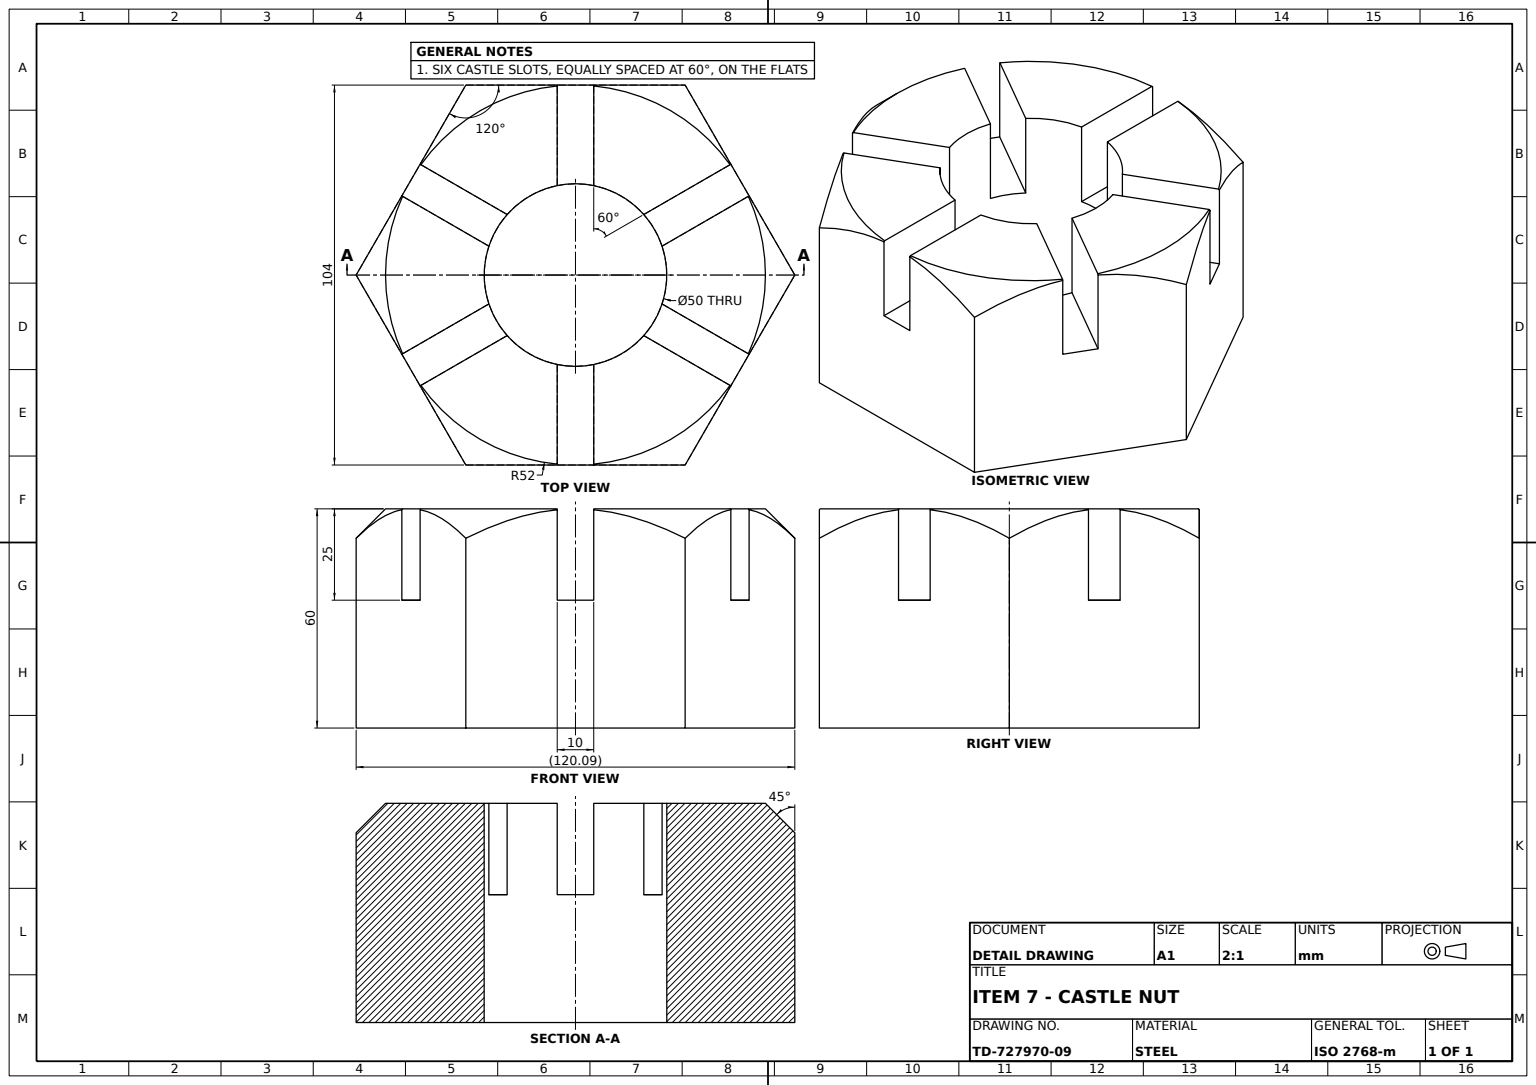
ISO-10303-21;
HEADER;
FILE_DESCRIPTION((''),'2;1');
FILE_NAME('','',(''),(''),'','','');
FILE_SCHEMA(('AUTOMOTIVE_DESIGN'));
ENDSEC;
DATA;
#1=APPLICATION_CONTEXT('');
#2=PRODUCT_CONTEXT('',#1,'mechanical');
#3=PRODUCT('','','',(#2));
#4=PRODUCT_DEFINITION_FORMATION('','',#3);
#5=PRODUCT_DEFINITION_CONTEXT('',#1,'design');
#6=PRODUCT_DEFINITION('','',#4,#5);
#7=PRODUCT_DEFINITION_SHAPE('','',#6);
#8=(LENGTH_UNIT()NAMED_UNIT(*)SI_UNIT(.MILLI.,.METRE.));
#9=(NAMED_UNIT(*)PLANE_ANGLE_UNIT()SI_UNIT($,.RADIAN.));
#10=(NAMED_UNIT(*)SI_UNIT($,.STERADIAN.)SOLID_ANGLE_UNIT());
#11=UNCERTAINTY_MEASURE_WITH_UNIT(LENGTH_MEASURE(1.E-05),#8,'distance_accuracy_value','');
#12=(GEOMETRIC_REPRESENTATION_CONTEXT(3)GLOBAL_UNCERTAINTY_ASSIGNED_CONTEXT((#11))GLOBAL_UNIT_ASSIGNED_CONTEXT((#8,#9,#10))REPRESENTATION_CONTEXT('',''));
#13=CARTESIAN_POINT('',(-23.713203,35.,-7.917322));
#14=VERTEX_POINT('',#13);
#15=CARTESIAN_POINT('',(-23.713203,60.,-7.917322));
#16=VERTEX_POINT('',#15);
#17=DIRECTION('',(0.,1.,0.));
#18=VECTOR('',#17,1000.);
#19=LINE('',#13,#18);
#20=EDGE_CURVE('',#14,#16,#19,.T.);
#21=ORIENTED_EDGE('',*,*,#20,.T.);
#22=CARTESIAN_POINT('',(-23.713203,60.,7.917322));
#23=VERTEX_POINT('',#22);
#24=CARTESIAN_POINT('',(0.,60.,0.));
#25=DIRECTION('',(0.,0.,1.));
#26=AXIS2_PLACEMENT_3D('',#24,#17,#25);
#27=CIRCLE('',#26,25.);
#28=EDGE_CURVE('',#16,#23,#27,.T.);
#29=ORIENTED_EDGE('',*,*,#28,.T.);
#30=CARTESIAN_POINT('',(-23.713203,35.,7.917322));
#31=VERTEX_POINT('',#30);
#32=LINE('',#30,#18);
#33=EDGE_CURVE('',#31,#23,#32,.T.);
#34=ORIENTED_EDGE('',*,*,#33,.F.);
#35=CARTESIAN_POINT('',(-18.713203,35.,16.577576));
#36=VERTEX_POINT('',#35);
#37=CARTESIAN_POINT('',(0.,35.,0.));
#38=DIRECTION('',(0.,-1.,0.));
#39=AXIS2_PLACEMENT_3D('',#37,#38,#25);
#40=CIRCLE('',#39,25.);
#41=EDGE_CURVE('',#36,#31,#40,.T.);
#42=ORIENTED_EDGE('',*,*,#41,.F.);
#43=CARTESIAN_POINT('',(-18.713203,60.,16.577576));
#44=VERTEX_POINT('',#43);
#45=LINE('',#35,#18);
#46=EDGE_CURVE('',#36,#44,#45,.T.);
#47=ORIENTED_EDGE('',*,*,#46,.T.);
#48=CARTESIAN_POINT('',(-5.,60.,24.494897));
#49=VERTEX_POINT('',#48);
#50=EDGE_CURVE('',#44,#49,#27,.T.);
#51=ORIENTED_EDGE('',*,*,#50,.T.);
#52=CARTESIAN_POINT('',(-5.,35.,24.494897));
#53=VERTEX_POINT('',#52);
#54=LINE('',#52,#18);
#55=EDGE_CURVE('',#53,#49,#54,.T.);
#56=ORIENTED_EDGE('',*,*,#55,.F.);
#57=CARTESIAN_POINT('',(0.,35.,25.));
#58=VERTEX_POINT('',#57);
#59=EDGE_CURVE('',#58,#53,#40,.T.);
#60=ORIENTED_EDGE('',*,*,#59,.F.);
#61=CARTESIAN_POINT('',(0.,0.,25.));
#62=VERTEX_POINT('',#61);
#63=LINE('',#61,#18);
#64=EDGE_CURVE('',#62,#58,#63,.T.);
#65=ORIENTED_EDGE('',*,*,#64,.F.);
#66=CARTESIAN_POINT('',(0.,0.,-25.));
#67=VERTEX_POINT('',#66);
#68=CARTESIAN_POINT('',(0.,0.,0.));
#69=AXIS2_PLACEMENT_3D('',#68,#17,#25);
#70=CIRCLE('',#69,25.);
#71=EDGE_CURVE('',#67,#62,#70,.T.);
#72=ORIENTED_EDGE('',*,*,#71,.F.);
#73=CARTESIAN_POINT('',(0.,35.,-25.));
#74=VERTEX_POINT('',#73);
#75=LINE('',#66,#18);
#76=EDGE_CURVE('',#67,#74,#75,.T.);
#77=ORIENTED_EDGE('',*,*,#76,.T.);
#78=CARTESIAN_POINT('',(-5.,35.,-24.494897));
#79=VERTEX_POINT('',#78);
#80=EDGE_CURVE('',#79,#74,#40,.T.);
#81=ORIENTED_EDGE('',*,*,#80,.F.);
#82=CARTESIAN_POINT('',(-5.,60.,-24.494897));
#83=VERTEX_POINT('',#82);
#84=LINE('',#78,#18);
#85=EDGE_CURVE('',#79,#83,#84,.T.);
#86=ORIENTED_EDGE('',*,*,#85,.T.);
#87=CARTESIAN_POINT('',(-18.713203,60.,-16.577576));
#88=VERTEX_POINT('',#87);
#89=EDGE_CURVE('',#83,#88,#27,.T.);
#90=ORIENTED_EDGE('',*,*,#89,.T.);
#91=CARTESIAN_POINT('',(-18.713203,35.,-16.577576));
#92=VERTEX_POINT('',#91);
#93=LINE('',#91,#18);
#94=EDGE_CURVE('',#92,#88,#93,.T.);
#95=ORIENTED_EDGE('',*,*,#94,.F.);
#96=EDGE_CURVE('',#14,#92,#40,.T.);
#97=ORIENTED_EDGE('',*,*,#96,.F.);
#98=EDGE_LOOP('',(#21,#29,#34,#42,#47,#51,#56,#60,#65,#72,#77,#81,#86,#90,#95,#97));
#99=FACE_OUTER_BOUND('',#98,.T.);
#100=CYLINDRICAL_SURFACE('',#69,25.);
#101=ADVANCED_FACE('',(#99),#100,.F.);
#102=CARTESIAN_POINT('',(23.713203,35.,-7.917322));
#103=VERTEX_POINT('',#102);
#104=CARTESIAN_POINT('',(47.533321,35.,-21.669873));
#105=VERTEX_POINT('',#104);
#106=DIRECTION('',(0.866025404,0.,-0.5));
#107=VECTOR('',#106,1000.);
#108=LINE('',#102,#107);
#109=EDGE_CURVE('',#103,#105,#108,.T.);
#110=ORIENTED_EDGE('',*,*,#109,.F.);
#111=CARTESIAN_POINT('',(23.713203,60.,-7.917322));
#112=VERTEX_POINT('',#111);
#113=LINE('',#102,#18);
#114=EDGE_CURVE('',#103,#112,#113,.T.);
#115=ORIENTED_EDGE('',*,*,#114,.T.);
#116=CARTESIAN_POINT('',(47.324658,60.,-21.549402));
#117=VERTEX_POINT('',#116);
#118=LINE('',#111,#107);
#119=EDGE_CURVE('',#112,#117,#118,.T.);
#120=ORIENTED_EDGE('',*,*,#119,.T.);
#121=CARTESIAN_POINT('',(47.533321,59.760168,-21.669873));
#122=VERTEX_POINT('',#121);
#123=CARTESIAN_POINT('',(47.394213,59.920057,-21.589559));
#124=CARTESIAN_POINT('',(47.463768,59.840113,-21.629716));
#125=B_SPLINE_CURVE_WITH_KNOTS('',3,(#116,#123,#124,#121),.UNSPECIFIED.,.F.,.F.,(4,4),(0.000000284,0.000340243),.UNSPECIFIED.);
#126=EDGE_CURVE('',#117,#122,#125,.T.);
#127=ORIENTED_EDGE('',*,*,#126,.T.);
#128=LINE('',#104,#18);
#129=EDGE_CURVE('',#105,#122,#128,.T.);
#130=ORIENTED_EDGE('',*,*,#129,.F.);
#131=EDGE_LOOP('',(#110,#115,#120,#127,#130));
#132=FACE_OUTER_BOUND('',#131,.T.);
#133=DIRECTION('',(0.5,0.,0.866025404));
#134=AXIS2_PLACEMENT_3D('',#102,#133,#106);
#135=PLANE('',#134);
#136=ADVANCED_FACE('',(#132),#135,.F.);
#137=CARTESIAN_POINT('',(-5.,35.,-52.));
#138=VERTEX_POINT('',#137);
#139=VECTOR('',#25,1000.);
#140=LINE('',#78,#139);
#141=EDGE_CURVE('',#138,#79,#140,.T.);
#142=ORIENTED_EDGE('',*,*,#141,.T.);
#143=ORIENTED_EDGE('',*,*,#80,.T.);
#144=CARTESIAN_POINT('',(5.,35.,-24.494897));
#145=VERTEX_POINT('',#144);
#146=EDGE_CURVE('',#74,#145,#40,.T.);
#147=ORIENTED_EDGE('',*,*,#146,.T.);
#148=CARTESIAN_POINT('',(5.,35.,-52.));
#149=VERTEX_POINT('',#148);
#150=DIRECTION('',(0.,0.,-1.));
#151=VECTOR('',#150,1000.);
#152=LINE('',#144,#151);
#153=EDGE_CURVE('',#145,#149,#152,.T.);
#154=ORIENTED_EDGE('',*,*,#153,.T.);
#155=DIRECTION('',(-1.,0.,0.));
#156=VECTOR('',#155,1000.);
#157=LINE('',#148,#156);
#158=EDGE_CURVE('',#149,#138,#157,.T.);
#159=ORIENTED_EDGE('',*,*,#158,.T.);
#160=EDGE_LOOP('',(#142,#143,#147,#154,#159));
#161=FACE_OUTER_BOUND('',#160,.T.);
#162=AXIS2_PLACEMENT_3D('',#37,#17,#25);
#163=PLANE('',#162);
#164=ADVANCED_FACE('',(#161),#163,.T.);
#165=CARTESIAN_POINT('',(-42.324658,60.,-30.209656));
#166=VERTEX_POINT('',#165);
#167=DIRECTION('',(-0.866025404,0.,-0.5));
#168=VECTOR('',#167,1000.);
#169=LINE('',#87,#168);
#170=EDGE_CURVE('',#88,#166,#169,.T.);
#171=ORIENTED_EDGE('',*,*,#170,.T.);
#172=CARTESIAN_POINT('',(-42.533321,59.760168,-30.330127));
#173=VERTEX_POINT('',#172);
#174=CARTESIAN_POINT('',(-42.394213,59.920057,-30.249813));
#175=CARTESIAN_POINT('',(-42.463768,59.840113,-30.28997));
#176=B_SPLINE_CURVE_WITH_KNOTS('',3,(#165,#174,#175,#172),.UNSPECIFIED.,.F.,.F.,(4,4),(0.000000284,0.000340243),.UNSPECIFIED.);
#177=EDGE_CURVE('',#166,#173,#176,.T.);
#178=ORIENTED_EDGE('',*,*,#177,.T.);
#179=CARTESIAN_POINT('',(-42.533321,35.,-30.330127));
#180=VERTEX_POINT('',#179);
#181=LINE('',#179,#18);
#182=EDGE_CURVE('',#180,#173,#181,.T.);
#183=ORIENTED_EDGE('',*,*,#182,.F.);
#184=LINE('',#91,#168);
#185=EDGE_CURVE('',#92,#180,#184,.T.);
#186=ORIENTED_EDGE('',*,*,#185,.F.);
#187=ORIENTED_EDGE('',*,*,#94,.T.);
#188=EDGE_LOOP('',(#171,#178,#183,#186,#187));
#189=FACE_OUTER_BOUND('',#188,.T.);
#190=DIRECTION('',(0.5,0.,-0.866025404));
#191=AXIS2_PLACEMENT_3D('',#91,#190,#167);
#192=PLANE('',#191);
#193=ADVANCED_FACE('',(#189),#192,.F.);
#194=CARTESIAN_POINT('',(18.713203,35.,16.577576));
#195=VERTEX_POINT('',#194);
#196=CARTESIAN_POINT('',(18.713203,60.,16.577576));
#197=VERTEX_POINT('',#196);
#198=LINE('',#194,#18);
#199=EDGE_CURVE('',#195,#197,#198,.T.);
#200=ORIENTED_EDGE('',*,*,#199,.T.);
#201=CARTESIAN_POINT('',(42.324658,60.,30.209656));
#202=VERTEX_POINT('',#201);
#203=DIRECTION('',(0.866025404,0.,0.5));
#204=VECTOR('',#203,1000.);
#205=LINE('',#196,#204);
#206=EDGE_CURVE('',#197,#202,#205,.T.);
#207=ORIENTED_EDGE('',*,*,#206,.T.);
#208=CARTESIAN_POINT('',(42.533321,59.760168,30.330127));
#209=VERTEX_POINT('',#208);
#210=CARTESIAN_POINT('',(42.394213,59.920057,30.249813));
#211=CARTESIAN_POINT('',(42.463768,59.840113,30.28997));
#212=B_SPLINE_CURVE_WITH_KNOTS('',3,(#201,#210,#211,#208),.UNSPECIFIED.,.F.,.F.,(4,4),(0.000000284,0.000340243),.UNSPECIFIED.);
#213=EDGE_CURVE('',#202,#209,#212,.T.);
#214=ORIENTED_EDGE('',*,*,#213,.T.);
#215=CARTESIAN_POINT('',(42.533321,35.,30.330127));
#216=VERTEX_POINT('',#215);
#217=LINE('',#215,#18);
#218=EDGE_CURVE('',#216,#209,#217,.T.);
#219=ORIENTED_EDGE('',*,*,#218,.F.);
#220=LINE('',#194,#204);
#221=EDGE_CURVE('',#195,#216,#220,.T.);
#222=ORIENTED_EDGE('',*,*,#221,.F.);
#223=EDGE_LOOP('',(#200,#207,#214,#219,#222));
#224=FACE_OUTER_BOUND('',#223,.T.);
#225=DIRECTION('',(-0.5,0.,0.866025404));
#226=AXIS2_PLACEMENT_3D('',#194,#225,#203);
#227=PLANE('',#226);
#228=ADVANCED_FACE('',(#224),#227,.F.);
#229=CARTESIAN_POINT('',(-5.,60.,-51.759057));
#230=VERTEX_POINT('',#229);
#231=LINE('',#82,#139);
#232=EDGE_CURVE('',#230,#83,#231,.T.);
#233=ORIENTED_EDGE('',*,*,#232,.T.);
#234=ORIENTED_EDGE('',*,*,#85,.F.);
#235=ORIENTED_EDGE('',*,*,#141,.F.);
#236=CARTESIAN_POINT('',(-5.,59.760168,-52.));
#237=VERTEX_POINT('',#236);
#238=LINE('',#137,#18);
#239=EDGE_CURVE('',#138,#237,#238,.T.);
#240=ORIENTED_EDGE('',*,*,#239,.T.);
#241=CARTESIAN_POINT('',(-5.,59.840113,-51.919687));
#242=CARTESIAN_POINT('',(-5.,59.920057,-51.839372));
#243=B_SPLINE_CURVE_WITH_KNOTS('',3,(#236,#241,#242,#229),.UNSPECIFIED.,.F.,.F.,(4,4),(0.041725978,0.042065937),.UNSPECIFIED.);
#244=EDGE_CURVE('',#237,#230,#243,.T.);
#245=ORIENTED_EDGE('',*,*,#244,.T.);
#246=EDGE_LOOP('',(#233,#234,#235,#240,#245));
#247=FACE_OUTER_BOUND('',#246,.T.);
#248=AXIS2_PLACEMENT_3D('',#78,#155,#25);
#249=PLANE('',#248);
#250=ADVANCED_FACE('',(#247),#249,.F.);
#251=CARTESIAN_POINT('',(60.044428,51.955572,0.));
#252=VERTEX_POINT('',#251);
#253=CARTESIAN_POINT('',(58.061924,53.938076,-3.433798));
#254=CARTESIAN_POINT('',(56.041415,55.66825,-6.933422));
#255=CARTESIAN_POINT('',(51.885852,58.368085,-14.131069));
#256=CARTESIAN_POINT('',(49.750496,59.335746,-17.829613));
#257=B_SPLINE_CURVE_WITH_KNOTS('',3,(#251,#253,#254,#255,#256,#121),.UNSPECIFIED.,.F.,.F.,(4,2,4),(0.000000254,0.013105191,0.026210128),.UNSPECIFIED.);
#258=EDGE_CURVE('',#252,#122,#257,.T.);
#259=ORIENTED_EDGE('',*,*,#258,.F.);
#260=CARTESIAN_POINT('',(60.044428,0.,0.));
#261=VERTEX_POINT('',#260);
#262=CARTESIAN_POINT('',(60.044428,60.,0.));
#263=VECTOR('',#38,1000.);
#264=LINE('',#262,#263);
#265=EDGE_CURVE('',#252,#261,#264,.T.);
#266=ORIENTED_EDGE('',*,*,#265,.T.);
#267=CARTESIAN_POINT('',(30.022214,0.,-52.));
#268=VERTEX_POINT('',#267);
#269=DIRECTION('',(-0.5,0.,-0.866025404));
#270=VECTOR('',#269,1000.);
#271=LINE('',#260,#270);
#272=EDGE_CURVE('',#261,#268,#271,.T.);
#273=ORIENTED_EDGE('',*,*,#272,.T.);
#274=CARTESIAN_POINT('',(30.022214,51.955572,-52.));
#275=VERTEX_POINT('',#274);
#276=CARTESIAN_POINT('',(30.022214,60.,-52.));
#277=LINE('',#276,#263);
#278=EDGE_CURVE('',#275,#268,#277,.T.);
#279=ORIENTED_EDGE('',*,*,#278,.F.);
#280=CARTESIAN_POINT('',(42.533321,59.760168,-30.330127));
#281=VERTEX_POINT('',#280);
#282=CARTESIAN_POINT('',(41.448793,59.552563,-32.208585));
#283=CARTESIAN_POINT('',(40.371647,59.212181,-34.074256));
#284=CARTESIAN_POINT('',(38.765983,58.520795,-36.855348));
#285=CARTESIAN_POINT('',(38.232434,58.26026,-37.779482));
#286=CARTESIAN_POINT('',(37.168479,57.682651,-39.622306));
#287=CARTESIAN_POINT('',(36.638429,57.365636,-40.54038));
#288=CARTESIAN_POINT('',(35.066096,56.345261,-43.26374));
#289=CARTESIAN_POINT('',(34.036763,55.570343,-45.046597));
#290=CARTESIAN_POINT('',(32.008326,53.869018,-48.559953));
#291=CARTESIAN_POINT('',(31.009226,52.942584,-50.290445));
#292=B_SPLINE_CURVE_WITH_KNOTS('',3,(#280,#282,#283,#284,#285,#286,#287,#288,#289,#290,#291,#274),.UNSPECIFIED.,.F.,.F.,(4,2,2,2,2,4),(0.036078749,0.042565008,0.045808138,0.049051268,0.055537527,0.062023787),.UNSPECIFIED.);
#293=EDGE_CURVE('',#281,#275,#292,.T.);
#294=ORIENTED_EDGE('',*,*,#293,.F.);
#295=CARTESIAN_POINT('',(42.533321,35.,-30.330127));
#296=VERTEX_POINT('',#295);
#297=LINE('',#295,#18);
#298=EDGE_CURVE('',#296,#281,#297,.T.);
#299=ORIENTED_EDGE('',*,*,#298,.F.);
#300=LINE('',#104,#270);
#301=EDGE_CURVE('',#105,#296,#300,.T.);
#302=ORIENTED_EDGE('',*,*,#301,.F.);
#303=ORIENTED_EDGE('',*,*,#129,.T.);
#304=EDGE_LOOP('',(#259,#266,#273,#279,#294,#299,#302,#303));
#305=FACE_OUTER_BOUND('',#304,.T.);
#306=DIRECTION('',(-0.866025404,0.,0.5));
#307=AXIS2_PLACEMENT_3D('',#262,#306,#133);
#308=PLANE('',#307);
#309=ADVANCED_FACE('',(#305),#308,.F.);
#310=ORIENTED_EDGE('',*,*,#119,.F.);
#311=CARTESIAN_POINT('',(23.713203,60.,7.917322));
#312=VERTEX_POINT('',#311);
#313=EDGE_CURVE('',#312,#112,#27,.T.);
#314=ORIENTED_EDGE('',*,*,#313,.F.);
#315=CARTESIAN_POINT('',(47.324658,60.,21.549402));
#316=VERTEX_POINT('',#315);
#317=LINE('',#311,#168);
#318=EDGE_CURVE('',#316,#312,#317,.T.);
#319=ORIENTED_EDGE('',*,*,#318,.F.);
#320=CIRCLE('',#26,52.);
#321=EDGE_CURVE('',#316,#117,#320,.T.);
#322=ORIENTED_EDGE('',*,*,#321,.T.);
#323=EDGE_LOOP('',(#310,#314,#319,#322));
#324=FACE_OUTER_BOUND('',#323,.T.);
#325=PLANE('',#26);
#326=ADVANCED_FACE('',(#324),#325,.T.);
#327=CARTESIAN_POINT('',(-47.533321,35.,21.669873));
#328=VERTEX_POINT('',#327);
#329=VECTOR('',#306,1000.);
#330=LINE('',#30,#329);
#331=EDGE_CURVE('',#31,#328,#330,.T.);
#332=ORIENTED_EDGE('',*,*,#331,.F.);
#333=ORIENTED_EDGE('',*,*,#33,.T.);
#334=CARTESIAN_POINT('',(-47.324658,60.,21.549402));
#335=VERTEX_POINT('',#334);
#336=LINE('',#22,#329);
#337=EDGE_CURVE('',#23,#335,#336,.T.);
#338=ORIENTED_EDGE('',*,*,#337,.T.);
#339=CARTESIAN_POINT('',(-47.533321,59.760168,21.669873));
#340=VERTEX_POINT('',#339);
#341=CARTESIAN_POINT('',(-47.394213,59.920057,21.589559));
#342=CARTESIAN_POINT('',(-47.463768,59.840113,21.629716));
#343=B_SPLINE_CURVE_WITH_KNOTS('',3,(#334,#341,#342,#339),.UNSPECIFIED.,.F.,.F.,(4,4),(0.000000284,0.000340243),.UNSPECIFIED.);
#344=EDGE_CURVE('',#335,#340,#343,.T.);
#345=ORIENTED_EDGE('',*,*,#344,.T.);
#346=LINE('',#327,#18);
#347=EDGE_CURVE('',#328,#340,#346,.T.);
#348=ORIENTED_EDGE('',*,*,#347,.F.);
#349=EDGE_LOOP('',(#332,#333,#338,#345,#348));
#350=FACE_OUTER_BOUND('',#349,.T.);
#351=AXIS2_PLACEMENT_3D('',#30,#269,#306);
#352=PLANE('',#351);
#353=ADVANCED_FACE('',(#350),#352,.F.);
#354=CARTESIAN_POINT('',(-5.,60.,51.759057));
#355=VERTEX_POINT('',#354);
#356=CARTESIAN_POINT('',(-5.,59.760168,52.));
#357=VERTEX_POINT('',#356);
#358=CARTESIAN_POINT('',(-5.,59.920057,51.839372));
#359=CARTESIAN_POINT('',(-5.,59.840113,51.919687));
#360=B_SPLINE_CURVE_WITH_KNOTS('',3,(#354,#358,#359,#356),.UNSPECIFIED.,.F.,.F.,(4,4),(0.039862447,0.040202405),.UNSPECIFIED.);
#361=EDGE_CURVE('',#355,#357,#360,.T.);
#362=ORIENTED_EDGE('',*,*,#361,.F.);
#363=CARTESIAN_POINT('',(-42.324658,60.,30.209656));
#364=VERTEX_POINT('',#363);
#365=EDGE_CURVE('',#364,#355,#320,.T.);
#366=ORIENTED_EDGE('',*,*,#365,.F.);
#367=CARTESIAN_POINT('',(-42.533321,59.760168,30.330127));
#368=VERTEX_POINT('',#367);
#369=CARTESIAN_POINT('',(-42.463768,59.840113,30.28997));
#370=CARTESIAN_POINT('',(-42.394213,59.920057,30.249813));
#371=B_SPLINE_CURVE_WITH_KNOTS('',3,(#367,#369,#370,#363),.UNSPECIFIED.,.F.,.F.,(4,4),(0.000000326,0.000340286),.UNSPECIFIED.);
#372=EDGE_CURVE('',#368,#364,#371,.T.);
#373=ORIENTED_EDGE('',*,*,#372,.F.);
#374=CARTESIAN_POINT('',(-30.022214,51.955572,52.));
#375=VERTEX_POINT('',#374);
#376=CARTESIAN_POINT('',(-41.448793,59.552563,32.208585));
#377=CARTESIAN_POINT('',(-40.371647,59.212181,34.074256));
#378=CARTESIAN_POINT('',(-38.765983,58.520795,36.855348));
#379=CARTESIAN_POINT('',(-38.232434,58.26026,37.779482));
#380=CARTESIAN_POINT('',(-37.168479,57.682651,39.622306));
#381=CARTESIAN_POINT('',(-36.638429,57.365636,40.54038));
#382=CARTESIAN_POINT('',(-35.066096,56.345261,43.26374));
#383=CARTESIAN_POINT('',(-34.036763,55.570343,45.046597));
#384=CARTESIAN_POINT('',(-32.008326,53.869018,48.559953));
#385=CARTESIAN_POINT('',(-31.009226,52.942584,50.290445));
#386=B_SPLINE_CURVE_WITH_KNOTS('',3,(#367,#376,#377,#378,#379,#380,#381,#382,#383,#384,#385,#374),.UNSPECIFIED.,.F.,.F.,(4,2,2,2,2,4),(0.036078749,0.042565008,0.045808138,0.049051268,0.055537527,0.062023787),.UNSPECIFIED.);
#387=EDGE_CURVE('',#368,#375,#386,.T.);
#388=ORIENTED_EDGE('',*,*,#387,.T.);
#389=CARTESIAN_POINT('',(-26.087238,53.92306,52.));
#390=CARTESIAN_POINT('',(-22.058836,55.652787,52.));
#391=CARTESIAN_POINT('',(-16.840607,57.349913,52.));
#392=CARTESIAN_POINT('',(-15.787712,57.665799,52.));
#393=CARTESIAN_POINT('',(-13.661318,58.245138,52.));
#394=CARTESIAN_POINT('',(-12.584869,58.509193,52.));
#395=CARTESIAN_POINT('',(-9.34409,59.209262,52.));
#396=CARTESIAN_POINT('',(-7.176093,59.551889,52.));
#397=B_SPLINE_CURVE_WITH_KNOTS('',3,(#374,#389,#390,#391,#392,#393,#394,#395,#396,#356),.UNSPECIFIED.,.F.,.F.,(4,2,2,2,4),(0.102670522,0.115841936,0.11913479,0.122427644,0.129013351),.UNSPECIFIED.);
#398=EDGE_CURVE('',#375,#357,#397,.T.);
#399=ORIENTED_EDGE('',*,*,#398,.T.);
#400=EDGE_LOOP('',(#362,#366,#373,#388,#399));
#401=FACE_OUTER_BOUND('',#400,.T.);
#402=AXIS2_PLACEMENT_3D('',#24,#38,#25);
#403=CONICAL_SURFACE('',#402,52.,0.785398163);
#404=ADVANCED_FACE('',(#401),#403,.T.);
#405=EDGE_CURVE('',#230,#166,#320,.T.);
#406=ORIENTED_EDGE('',*,*,#405,.T.);
#407=ORIENTED_EDGE('',*,*,#170,.F.);
#408=ORIENTED_EDGE('',*,*,#89,.F.);
#409=ORIENTED_EDGE('',*,*,#232,.F.);
#410=EDGE_LOOP('',(#406,#407,#408,#409));
#411=FACE_OUTER_BOUND('',#410,.T.);
#412=ADVANCED_FACE('',(#411),#325,.T.);
#413=CARTESIAN_POINT('',(18.713203,35.,-16.577576));
#414=VERTEX_POINT('',#413);
#415=EDGE_CURVE('',#414,#103,#40,.T.);
#416=ORIENTED_EDGE('',*,*,#415,.T.);
#417=ORIENTED_EDGE('',*,*,#109,.T.);
#418=ORIENTED_EDGE('',*,*,#301,.T.);
#419=LINE('',#413,#329);
#420=EDGE_CURVE('',#296,#414,#419,.T.);
#421=ORIENTED_EDGE('',*,*,#420,.T.);
#422=EDGE_LOOP('',(#416,#417,#418,#421));
#423=FACE_OUTER_BOUND('',#422,.T.);
#424=ADVANCED_FACE('',(#423),#163,.T.);
#425=ORIENTED_EDGE('',*,*,#64,.T.);
#426=CARTESIAN_POINT('',(5.,35.,24.494897));
#427=VERTEX_POINT('',#426);
#428=EDGE_CURVE('',#427,#58,#40,.T.);
#429=ORIENTED_EDGE('',*,*,#428,.F.);
#430=CARTESIAN_POINT('',(5.,60.,24.494897));
#431=VERTEX_POINT('',#430);
#432=LINE('',#426,#18);
#433=EDGE_CURVE('',#427,#431,#432,.T.);
#434=ORIENTED_EDGE('',*,*,#433,.T.);
#435=EDGE_CURVE('',#431,#197,#27,.T.);
#436=ORIENTED_EDGE('',*,*,#435,.T.);
#437=ORIENTED_EDGE('',*,*,#199,.F.);
#438=CARTESIAN_POINT('',(23.713203,35.,7.917322));
#439=VERTEX_POINT('',#438);
#440=EDGE_CURVE('',#439,#195,#40,.T.);
#441=ORIENTED_EDGE('',*,*,#440,.F.);
#442=LINE('',#438,#18);
#443=EDGE_CURVE('',#439,#312,#442,.T.);
#444=ORIENTED_EDGE('',*,*,#443,.T.);
#445=ORIENTED_EDGE('',*,*,#313,.T.);
#446=ORIENTED_EDGE('',*,*,#114,.F.);
#447=ORIENTED_EDGE('',*,*,#415,.F.);
#448=CARTESIAN_POINT('',(18.713203,60.,-16.577576));
#449=VERTEX_POINT('',#448);
#450=LINE('',#413,#18);
#451=EDGE_CURVE('',#414,#449,#450,.T.);
#452=ORIENTED_EDGE('',*,*,#451,.T.);
#453=CARTESIAN_POINT('',(5.,60.,-24.494897));
#454=VERTEX_POINT('',#453);
#455=EDGE_CURVE('',#449,#454,#27,.T.);
#456=ORIENTED_EDGE('',*,*,#455,.T.);
#457=LINE('',#144,#18);
#458=EDGE_CURVE('',#145,#454,#457,.T.);
#459=ORIENTED_EDGE('',*,*,#458,.F.);
#460=ORIENTED_EDGE('',*,*,#146,.F.);
#461=ORIENTED_EDGE('',*,*,#76,.F.);
#462=EDGE_CURVE('',#62,#67,#70,.T.);
#463=ORIENTED_EDGE('',*,*,#462,.F.);
#464=EDGE_LOOP('',(#425,#429,#434,#436,#437,#441,#444,#445,#446,#447,#452,#456,#459,#460,#461,#463));
#465=FACE_OUTER_BOUND('',#464,.T.);
#466=ADVANCED_FACE('',(#465),#100,.F.);
#467=CARTESIAN_POINT('',(-42.533321,35.,30.330127));
#468=VERTEX_POINT('',#467);
#469=LINE('',#35,#107);
#470=EDGE_CURVE('',#468,#36,#469,.T.);
#471=ORIENTED_EDGE('',*,*,#470,.F.);
#472=LINE('',#467,#18);
#473=EDGE_CURVE('',#468,#368,#472,.T.);
#474=ORIENTED_EDGE('',*,*,#473,.T.);
#475=ORIENTED_EDGE('',*,*,#372,.T.);
#476=LINE('',#43,#107);
#477=EDGE_CURVE('',#364,#44,#476,.T.);
#478=ORIENTED_EDGE('',*,*,#477,.T.);
#479=ORIENTED_EDGE('',*,*,#46,.F.);
#480=EDGE_LOOP('',(#471,#474,#475,#478,#479));
#481=FACE_OUTER_BOUND('',#480,.T.);
#482=AXIS2_PLACEMENT_3D('',#35,#133,#106);
#483=PLANE('',#482);
#484=ADVANCED_FACE('',(#481),#483,.F.);
#485=CARTESIAN_POINT('',(-47.533321,35.,-21.669873));
#486=VERTEX_POINT('',#485);
#487=CARTESIAN_POINT('',(-47.533321,59.760168,-21.669873));
#488=VERTEX_POINT('',#487);
#489=LINE('',#485,#18);
#490=EDGE_CURVE('',#486,#488,#489,.T.);
#491=ORIENTED_EDGE('',*,*,#490,.F.);
#492=VECTOR('',#225,1000.);
#493=LINE('',#179,#492);
#494=EDGE_CURVE('',#180,#486,#493,.T.);
#495=ORIENTED_EDGE('',*,*,#494,.F.);
#496=ORIENTED_EDGE('',*,*,#182,.T.);
#497=CARTESIAN_POINT('',(-30.022214,51.955572,-52.));
#498=VERTEX_POINT('',#497);
#499=CARTESIAN_POINT('',(-32.004718,53.938076,-48.566202));
#500=CARTESIAN_POINT('',(-34.025227,55.66825,-45.066578));
#501=CARTESIAN_POINT('',(-38.18079,58.368085,-37.868931));
#502=CARTESIAN_POINT('',(-40.316146,59.335746,-34.170387));
#503=B_SPLINE_CURVE_WITH_KNOTS('',3,(#497,#499,#500,#501,#502,#172),.UNSPECIFIED.,.F.,.F.,(4,2,4),(0.000000254,0.013105191,0.026210128),.UNSPECIFIED.);
#504=EDGE_CURVE('',#498,#173,#503,.T.);
#505=ORIENTED_EDGE('',*,*,#504,.F.);
#506=CARTESIAN_POINT('',(-30.022214,0.,-52.));
#507=VERTEX_POINT('',#506);
#508=CARTESIAN_POINT('',(-30.022214,60.,-52.));
#509=LINE('',#508,#263);
#510=EDGE_CURVE('',#498,#507,#509,.T.);
#511=ORIENTED_EDGE('',*,*,#510,.T.);
#512=CARTESIAN_POINT('',(-60.044428,0.,0.));
#513=VERTEX_POINT('',#512);
#514=LINE('',#506,#492);
#515=EDGE_CURVE('',#507,#513,#514,.T.);
#516=ORIENTED_EDGE('',*,*,#515,.T.);
#517=CARTESIAN_POINT('',(-60.044428,51.955572,0.));
#518=VERTEX_POINT('',#517);
#519=CARTESIAN_POINT('',(-60.044428,60.,0.));
#520=LINE('',#519,#263);
#521=EDGE_CURVE('',#518,#513,#520,.T.);
#522=ORIENTED_EDGE('',*,*,#521,.F.);
#523=CARTESIAN_POINT('',(-48.617849,59.552563,-19.791415));
#524=CARTESIAN_POINT('',(-49.694995,59.212181,-17.925744));
#525=CARTESIAN_POINT('',(-51.300659,58.520795,-15.144652));
#526=CARTESIAN_POINT('',(-51.834208,58.26026,-14.220518));
#527=CARTESIAN_POINT('',(-52.898163,57.682651,-12.377694));
#528=CARTESIAN_POINT('',(-53.428213,57.365636,-11.45962));
#529=CARTESIAN_POINT('',(-55.000546,56.345261,-8.73626));
#530=CARTESIAN_POINT('',(-56.029879,55.570343,-6.953403));
#531=CARTESIAN_POINT('',(-58.058316,53.869018,-3.440047));
#532=CARTESIAN_POINT('',(-59.057416,52.942584,-1.709555));
#533=B_SPLINE_CURVE_WITH_KNOTS('',3,(#487,#523,#524,#525,#526,#527,#528,#529,#530,#531,#532,#517),.UNSPECIFIED.,.F.,.F.,(4,2,2,2,2,4),(0.036078749,0.042565008,0.045808138,0.049051268,0.055537527,0.062023787),.UNSPECIFIED.);
#534=EDGE_CURVE('',#488,#518,#533,.T.);
#535=ORIENTED_EDGE('',*,*,#534,.F.);
#536=EDGE_LOOP('',(#491,#495,#496,#505,#511,#516,#522,#535));
#537=FACE_OUTER_BOUND('',#536,.T.);
#538=AXIS2_PLACEMENT_3D('',#508,#203,#190);
#539=PLANE('',#538);
#540=ADVANCED_FACE('',(#537),#539,.F.);
#541=ORIENTED_EDGE('',*,*,#428,.T.);
#542=ORIENTED_EDGE('',*,*,#59,.T.);
#543=CARTESIAN_POINT('',(-5.,35.,52.));
#544=VERTEX_POINT('',#543);
#545=LINE('',#52,#139);
#546=EDGE_CURVE('',#53,#544,#545,.T.);
#547=ORIENTED_EDGE('',*,*,#546,.T.);
#548=CARTESIAN_POINT('',(5.,35.,52.));
#549=VERTEX_POINT('',#548);
#550=DIRECTION('',(1.,0.,0.));
#551=VECTOR('',#550,1000.);
#552=LINE('',#543,#551);
#553=EDGE_CURVE('',#544,#549,#552,.T.);
#554=ORIENTED_EDGE('',*,*,#553,.T.);
#555=LINE('',#426,#151);
#556=EDGE_CURVE('',#549,#427,#555,.T.);
#557=ORIENTED_EDGE('',*,*,#556,.T.);
#558=EDGE_LOOP('',(#541,#542,#547,#554,#557));
#559=FACE_OUTER_BOUND('',#558,.T.);
#560=ADVANCED_FACE('',(#559),#163,.T.);
#561=ORIENTED_EDGE('',*,*,#546,.F.);
#562=ORIENTED_EDGE('',*,*,#55,.T.);
#563=LINE('',#48,#139);
#564=EDGE_CURVE('',#49,#355,#563,.T.);
#565=ORIENTED_EDGE('',*,*,#564,.T.);
#566=ORIENTED_EDGE('',*,*,#361,.T.);
#567=LINE('',#543,#18);
#568=EDGE_CURVE('',#544,#357,#567,.T.);
#569=ORIENTED_EDGE('',*,*,#568,.F.);
#570=EDGE_LOOP('',(#561,#562,#565,#566,#569));
#571=FACE_OUTER_BOUND('',#570,.T.);
#572=AXIS2_PLACEMENT_3D('',#52,#155,#25);
#573=PLANE('',#572);
#574=ADVANCED_FACE('',(#571),#573,.F.);
#575=ORIENTED_EDGE('',*,*,#405,.F.);
#576=ORIENTED_EDGE('',*,*,#244,.F.);
#577=CARTESIAN_POINT('',(-5.549576,59.707567,-52.));
#578=CARTESIAN_POINT('',(-6.100498,59.6462,-52.));
#579=CARTESIAN_POINT('',(-7.196966,59.507138,-52.));
#580=CARTESIAN_POINT('',(-8.835057,59.273996,-52.));
#581=CARTESIAN_POINT('',(-10.454038,58.96989,-52.));
#582=CARTESIAN_POINT('',(-13.668472,58.274309,-52.));
#583=CARTESIAN_POINT('',(-15.780082,57.694187,-52.));
#584=CARTESIAN_POINT('',(-18.908127,56.677809,-52.));
#585=CARTESIAN_POINT('',(-19.944242,56.314633,-52.));
#586=CARTESIAN_POINT('',(-22.004532,55.54394,-52.));
#587=CARTESIAN_POINT('',(-23.030224,55.135779,-52.));
#588=CARTESIAN_POINT('',(-26.080408,53.855514,-52.));
#589=CARTESIAN_POINT('',(-28.068686,52.932336,-52.));
#590=B_SPLINE_CURVE_WITH_KNOTS('',3,(#236,#577,#578,#579,#580,#581,#582,#583,#584,#585,#586,#587,#588,#589,#497),.UNSPECIFIED.,.F.,.F.,(4,2,1,2,2,2,2,4),(0.139043469,0.140687624,0.142331778,0.145620087,0.152196705,0.155485014,0.158773323,0.16534994),.UNSPECIFIED.);
#591=EDGE_CURVE('',#237,#498,#590,.T.);
#592=ORIENTED_EDGE('',*,*,#591,.T.);
#593=ORIENTED_EDGE('',*,*,#504,.T.);
#594=ORIENTED_EDGE('',*,*,#177,.F.);
#595=EDGE_LOOP('',(#575,#576,#592,#593,#594));
#596=FACE_OUTER_BOUND('',#595,.T.);
#597=ADVANCED_FACE('',(#596),#403,.T.);
#598=ORIENTED_EDGE('',*,*,#153,.F.);
#599=ORIENTED_EDGE('',*,*,#458,.T.);
#600=CARTESIAN_POINT('',(5.,60.,-51.759057));
#601=VERTEX_POINT('',#600);
#602=LINE('',#453,#151);
#603=EDGE_CURVE('',#454,#601,#602,.T.);
#604=ORIENTED_EDGE('',*,*,#603,.T.);
#605=CARTESIAN_POINT('',(5.,59.760168,-52.));
#606=VERTEX_POINT('',#605);
#607=CARTESIAN_POINT('',(5.,59.920057,-51.839372));
#608=CARTESIAN_POINT('',(5.,59.840113,-51.919687));
#609=B_SPLINE_CURVE_WITH_KNOTS('',3,(#600,#607,#608,#605),.UNSPECIFIED.,.F.,.F.,(4,4),(0.039862447,0.040202405),.UNSPECIFIED.);
#610=EDGE_CURVE('',#601,#606,#609,.T.);
#611=ORIENTED_EDGE('',*,*,#610,.T.);
#612=LINE('',#148,#18);
#613=EDGE_CURVE('',#149,#606,#612,.T.);
#614=ORIENTED_EDGE('',*,*,#613,.F.);
#615=EDGE_LOOP('',(#598,#599,#604,#611,#614));
#616=FACE_OUTER_BOUND('',#615,.T.);
#617=AXIS2_PLACEMENT_3D('',#144,#550,#150);
#618=PLANE('',#617);
#619=ADVANCED_FACE('',(#616),#618,.F.);
#620=ORIENTED_EDGE('',*,*,#206,.F.);
#621=ORIENTED_EDGE('',*,*,#435,.F.);
#622=CARTESIAN_POINT('',(5.,60.,51.759057));
#623=VERTEX_POINT('',#622);
#624=LINE('',#430,#151);
#625=EDGE_CURVE('',#623,#431,#624,.T.);
#626=ORIENTED_EDGE('',*,*,#625,.F.);
#627=EDGE_CURVE('',#623,#202,#320,.T.);
#628=ORIENTED_EDGE('',*,*,#627,.T.);
#629=EDGE_LOOP('',(#620,#621,#626,#628));
#630=FACE_OUTER_BOUND('',#629,.T.);
#631=ADVANCED_FACE('',(#630),#325,.T.);
#632=CARTESIAN_POINT('',(30.022214,51.955572,52.));
#633=VERTEX_POINT('',#632);
#634=CARTESIAN_POINT('',(32.004718,53.938076,48.566202));
#635=CARTESIAN_POINT('',(34.025227,55.66825,45.066578));
#636=CARTESIAN_POINT('',(38.18079,58.368085,37.868931));
#637=CARTESIAN_POINT('',(40.316146,59.335746,34.170387));
#638=B_SPLINE_CURVE_WITH_KNOTS('',3,(#632,#634,#635,#636,#637,#208),.UNSPECIFIED.,.F.,.F.,(4,2,4),(0.000000254,0.013105191,0.026210128),.UNSPECIFIED.);
#639=EDGE_CURVE('',#633,#209,#638,.T.);
#640=ORIENTED_EDGE('',*,*,#639,.F.);
#641=CARTESIAN_POINT('',(30.022214,0.,52.));
#642=VERTEX_POINT('',#641);
#643=CARTESIAN_POINT('',(30.022214,60.,52.));
#644=LINE('',#643,#263);
#645=EDGE_CURVE('',#633,#642,#644,.T.);
#646=ORIENTED_EDGE('',*,*,#645,.T.);
#647=VECTOR('',#190,1000.);
#648=LINE('',#641,#647);
#649=EDGE_CURVE('',#642,#261,#648,.T.);
#650=ORIENTED_EDGE('',*,*,#649,.T.);
#651=ORIENTED_EDGE('',*,*,#265,.F.);
#652=CARTESIAN_POINT('',(47.533321,59.760168,21.669873));
#653=VERTEX_POINT('',#652);
#654=CARTESIAN_POINT('',(48.617849,59.552563,19.791415));
#655=CARTESIAN_POINT('',(49.694995,59.212181,17.925744));
#656=CARTESIAN_POINT('',(51.300659,58.520795,15.144652));
#657=CARTESIAN_POINT('',(51.834208,58.26026,14.220518));
#658=CARTESIAN_POINT('',(52.898163,57.682651,12.377694));
#659=CARTESIAN_POINT('',(53.428213,57.365636,11.45962));
#660=CARTESIAN_POINT('',(55.000546,56.345261,8.73626));
#661=CARTESIAN_POINT('',(56.029879,55.570343,6.953403));
#662=CARTESIAN_POINT('',(58.058316,53.869018,3.440047));
#663=CARTESIAN_POINT('',(59.057416,52.942584,1.709555));
#664=B_SPLINE_CURVE_WITH_KNOTS('',3,(#652,#654,#655,#656,#657,#658,#659,#660,#661,#662,#663,#251),.UNSPECIFIED.,.F.,.F.,(4,2,2,2,2,4),(0.036078749,0.042565008,0.045808138,0.049051268,0.055537527,0.062023787),.UNSPECIFIED.);
#665=EDGE_CURVE('',#653,#252,#664,.T.);
#666=ORIENTED_EDGE('',*,*,#665,.F.);
#667=CARTESIAN_POINT('',(47.533321,35.,21.669873));
#668=VERTEX_POINT('',#667);
#669=LINE('',#667,#18);
#670=EDGE_CURVE('',#668,#653,#669,.T.);
#671=ORIENTED_EDGE('',*,*,#670,.F.);
#672=LINE('',#215,#647);
#673=EDGE_CURVE('',#216,#668,#672,.T.);
#674=ORIENTED_EDGE('',*,*,#673,.F.);
#675=ORIENTED_EDGE('',*,*,#218,.T.);
#676=EDGE_LOOP('',(#640,#646,#650,#651,#666,#671,#674,#675));
#677=FACE_OUTER_BOUND('',#676,.T.);
#678=AXIS2_PLACEMENT_3D('',#643,#167,#225);
#679=PLANE('',#678);
#680=ADVANCED_FACE('',(#677),#679,.F.);
#681=ORIENTED_EDGE('',*,*,#50,.F.);
#682=ORIENTED_EDGE('',*,*,#477,.F.);
#683=ORIENTED_EDGE('',*,*,#365,.T.);
#684=ORIENTED_EDGE('',*,*,#564,.F.);
#685=EDGE_LOOP('',(#681,#682,#683,#684));
#686=FACE_OUTER_BOUND('',#685,.T.);
#687=ADVANCED_FACE('',(#686),#325,.T.);
#688=ORIENTED_EDGE('',*,*,#318,.T.);
#689=ORIENTED_EDGE('',*,*,#443,.F.);
#690=LINE('',#438,#168);
#691=EDGE_CURVE('',#668,#439,#690,.T.);
#692=ORIENTED_EDGE('',*,*,#691,.F.);
#693=ORIENTED_EDGE('',*,*,#670,.T.);
#694=CARTESIAN_POINT('',(47.463768,59.840113,21.629716));
#695=CARTESIAN_POINT('',(47.394213,59.920057,21.589559));
#696=B_SPLINE_CURVE_WITH_KNOTS('',3,(#652,#694,#695,#315),.UNSPECIFIED.,.F.,.F.,(4,4),(0.000000326,0.000340286),.UNSPECIFIED.);
#697=EDGE_CURVE('',#653,#316,#696,.T.);
#698=ORIENTED_EDGE('',*,*,#697,.T.);
#699=EDGE_LOOP('',(#688,#689,#692,#693,#698));
#700=FACE_OUTER_BOUND('',#699,.T.);
#701=AXIS2_PLACEMENT_3D('',#438,#190,#167);
#702=PLANE('',#701);
#703=ADVANCED_FACE('',(#700),#702,.F.);
#704=ORIENTED_EDGE('',*,*,#613,.T.);
#705=CARTESIAN_POINT('',(26.087238,53.92306,-52.));
#706=CARTESIAN_POINT('',(22.058836,55.652787,-52.));
#707=CARTESIAN_POINT('',(16.840607,57.349913,-52.));
#708=CARTESIAN_POINT('',(15.787712,57.665799,-52.));
#709=CARTESIAN_POINT('',(13.661318,58.245138,-52.));
#710=CARTESIAN_POINT('',(12.584869,58.509193,-52.));
#711=CARTESIAN_POINT('',(9.34409,59.209262,-52.));
#712=CARTESIAN_POINT('',(7.176093,59.551889,-52.));
#713=B_SPLINE_CURVE_WITH_KNOTS('',3,(#274,#705,#706,#707,#708,#709,#710,#711,#712,#605),.UNSPECIFIED.,.F.,.F.,(4,2,2,2,4),(0.102670522,0.115841936,0.11913479,0.122427644,0.129013351),.UNSPECIFIED.);
#714=EDGE_CURVE('',#275,#606,#713,.T.);
#715=ORIENTED_EDGE('',*,*,#714,.F.);
#716=ORIENTED_EDGE('',*,*,#278,.T.);
#717=LINE('',#267,#156);
#718=EDGE_CURVE('',#268,#507,#717,.T.);
#719=ORIENTED_EDGE('',*,*,#718,.T.);
#720=ORIENTED_EDGE('',*,*,#510,.F.);
#721=ORIENTED_EDGE('',*,*,#591,.F.);
#722=ORIENTED_EDGE('',*,*,#239,.F.);
#723=ORIENTED_EDGE('',*,*,#158,.F.);
#724=EDGE_LOOP('',(#704,#715,#716,#719,#720,#721,#722,#723));
#725=FACE_OUTER_BOUND('',#724,.T.);
#726=AXIS2_PLACEMENT_3D('',#276,#25,#550);
#727=PLANE('',#726);
#728=ADVANCED_FACE('',(#725),#727,.F.);
#729=ORIENTED_EDGE('',*,*,#344,.F.);
#730=CARTESIAN_POINT('',(-47.324658,60.,-21.549402));
#731=VERTEX_POINT('',#730);
#732=EDGE_CURVE('',#731,#335,#320,.T.);
#733=ORIENTED_EDGE('',*,*,#732,.F.);
#734=CARTESIAN_POINT('',(-47.463768,59.840113,-21.629716));
#735=CARTESIAN_POINT('',(-47.394213,59.920057,-21.589559));
#736=B_SPLINE_CURVE_WITH_KNOTS('',3,(#487,#734,#735,#730),.UNSPECIFIED.,.F.,.F.,(4,4),(0.000000326,0.000340286),.UNSPECIFIED.);
#737=EDGE_CURVE('',#488,#731,#736,.T.);
#738=ORIENTED_EDGE('',*,*,#737,.F.);
#739=ORIENTED_EDGE('',*,*,#534,.T.);
#740=CARTESIAN_POINT('',(-58.061924,53.938076,3.433798));
#741=CARTESIAN_POINT('',(-56.041415,55.66825,6.933422));
#742=CARTESIAN_POINT('',(-51.885852,58.368085,14.131069));
#743=CARTESIAN_POINT('',(-49.750496,59.335746,17.829613));
#744=B_SPLINE_CURVE_WITH_KNOTS('',3,(#517,#740,#741,#742,#743,#339),.UNSPECIFIED.,.F.,.F.,(4,2,4),(0.000000254,0.013105191,0.026210128),.UNSPECIFIED.);
#745=EDGE_CURVE('',#518,#340,#744,.T.);
#746=ORIENTED_EDGE('',*,*,#745,.T.);
#747=EDGE_LOOP('',(#729,#733,#738,#739,#746));
#748=FACE_OUTER_BOUND('',#747,.T.);
#749=ADVANCED_FACE('',(#748),#403,.T.);
#750=ORIENTED_EDGE('',*,*,#126,.F.);
#751=ORIENTED_EDGE('',*,*,#321,.F.);
#752=ORIENTED_EDGE('',*,*,#697,.F.);
#753=ORIENTED_EDGE('',*,*,#665,.T.);
#754=ORIENTED_EDGE('',*,*,#258,.T.);
#755=EDGE_LOOP('',(#750,#751,#752,#753,#754));
#756=FACE_OUTER_BOUND('',#755,.T.);
#757=ADVANCED_FACE('',(#756),#403,.T.);
#758=ORIENTED_EDGE('',*,*,#625,.T.);
#759=ORIENTED_EDGE('',*,*,#433,.F.);
#760=ORIENTED_EDGE('',*,*,#556,.F.);
#761=CARTESIAN_POINT('',(5.,59.760168,52.));
#762=VERTEX_POINT('',#761);
#763=LINE('',#548,#18);
#764=EDGE_CURVE('',#549,#762,#763,.T.);
#765=ORIENTED_EDGE('',*,*,#764,.T.);
#766=CARTESIAN_POINT('',(5.,59.840113,51.919687));
#767=CARTESIAN_POINT('',(5.,59.920057,51.839372));
#768=B_SPLINE_CURVE_WITH_KNOTS('',3,(#761,#766,#767,#622),.UNSPECIFIED.,.F.,.F.,(4,4),(0.041725978,0.042065937),.UNSPECIFIED.);
#769=EDGE_CURVE('',#762,#623,#768,.T.);
#770=ORIENTED_EDGE('',*,*,#769,.T.);
#771=EDGE_LOOP('',(#758,#759,#760,#765,#770));
#772=FACE_OUTER_BOUND('',#771,.T.);
#773=AXIS2_PLACEMENT_3D('',#426,#550,#150);
#774=PLANE('',#773);
#775=ADVANCED_FACE('',(#772),#774,.F.);
#776=ORIENTED_EDGE('',*,*,#714,.T.);
#777=ORIENTED_EDGE('',*,*,#610,.F.);
#778=CARTESIAN_POINT('',(42.324658,60.,-30.209656));
#779=VERTEX_POINT('',#778);
#780=EDGE_CURVE('',#779,#601,#320,.T.);
#781=ORIENTED_EDGE('',*,*,#780,.F.);
#782=CARTESIAN_POINT('',(42.463768,59.840113,-30.28997));
#783=CARTESIAN_POINT('',(42.394213,59.920057,-30.249813));
#784=B_SPLINE_CURVE_WITH_KNOTS('',3,(#280,#782,#783,#778),.UNSPECIFIED.,.F.,.F.,(4,4),(0.000000326,0.000340286),.UNSPECIFIED.);
#785=EDGE_CURVE('',#281,#779,#784,.T.);
#786=ORIENTED_EDGE('',*,*,#785,.F.);
#787=ORIENTED_EDGE('',*,*,#293,.T.);
#788=EDGE_LOOP('',(#776,#777,#781,#786,#787));
#789=FACE_OUTER_BOUND('',#788,.T.);
#790=ADVANCED_FACE('',(#789),#403,.T.);
#791=LINE('',#13,#204);
#792=EDGE_CURVE('',#486,#14,#791,.T.);
#793=ORIENTED_EDGE('',*,*,#792,.F.);
#794=ORIENTED_EDGE('',*,*,#490,.T.);
#795=ORIENTED_EDGE('',*,*,#737,.T.);
#796=LINE('',#15,#204);
#797=EDGE_CURVE('',#731,#16,#796,.T.);
#798=ORIENTED_EDGE('',*,*,#797,.T.);
#799=ORIENTED_EDGE('',*,*,#20,.F.);
#800=EDGE_LOOP('',(#793,#794,#795,#798,#799));
#801=FACE_OUTER_BOUND('',#800,.T.);
#802=AXIS2_PLACEMENT_3D('',#13,#225,#203);
#803=PLANE('',#802);
#804=ADVANCED_FACE('',(#801),#803,.F.);
#805=CARTESIAN_POINT('',(5.549576,59.707567,52.));
#806=CARTESIAN_POINT('',(6.100498,59.6462,52.));
#807=CARTESIAN_POINT('',(7.196966,59.507138,52.));
#808=CARTESIAN_POINT('',(8.835057,59.273996,52.));
#809=CARTESIAN_POINT('',(10.454038,58.96989,52.));
#810=CARTESIAN_POINT('',(13.668472,58.274309,52.));
#811=CARTESIAN_POINT('',(15.780082,57.694187,52.));
#812=CARTESIAN_POINT('',(18.908127,56.677809,52.));
#813=CARTESIAN_POINT('',(19.944242,56.314633,52.));
#814=CARTESIAN_POINT('',(22.004532,55.54394,52.));
#815=CARTESIAN_POINT('',(23.030224,55.135779,52.));
#816=CARTESIAN_POINT('',(26.080408,53.855514,52.));
#817=CARTESIAN_POINT('',(28.068686,52.932336,52.));
#818=B_SPLINE_CURVE_WITH_KNOTS('',3,(#761,#805,#806,#807,#808,#809,#810,#811,#812,#813,#814,#815,#816,#817,#632),.UNSPECIFIED.,.F.,.F.,(4,2,1,2,2,2,2,4),(0.139043469,0.140687624,0.142331778,0.145620087,0.152196705,0.155485014,0.158773323,0.16534994),.UNSPECIFIED.);
#819=EDGE_CURVE('',#762,#633,#818,.T.);
#820=ORIENTED_EDGE('',*,*,#819,.T.);
#821=ORIENTED_EDGE('',*,*,#639,.T.);
#822=ORIENTED_EDGE('',*,*,#213,.F.);
#823=ORIENTED_EDGE('',*,*,#627,.F.);
#824=ORIENTED_EDGE('',*,*,#769,.F.);
#825=EDGE_LOOP('',(#820,#821,#822,#823,#824));
#826=FACE_OUTER_BOUND('',#825,.T.);
#827=ADVANCED_FACE('',(#826),#403,.T.);
#828=ORIENTED_EDGE('',*,*,#28,.F.);
#829=ORIENTED_EDGE('',*,*,#797,.F.);
#830=ORIENTED_EDGE('',*,*,#732,.T.);
#831=ORIENTED_EDGE('',*,*,#337,.F.);
#832=EDGE_LOOP('',(#828,#829,#830,#831));
#833=FACE_OUTER_BOUND('',#832,.T.);
#834=ADVANCED_FACE('',(#833),#325,.T.);
#835=LINE('',#448,#329);
#836=EDGE_CURVE('',#779,#449,#835,.T.);
#837=ORIENTED_EDGE('',*,*,#836,.T.);
#838=ORIENTED_EDGE('',*,*,#451,.F.);
#839=ORIENTED_EDGE('',*,*,#420,.F.);
#840=ORIENTED_EDGE('',*,*,#298,.T.);
#841=ORIENTED_EDGE('',*,*,#785,.T.);
#842=EDGE_LOOP('',(#837,#838,#839,#840,#841));
#843=FACE_OUTER_BOUND('',#842,.T.);
#844=AXIS2_PLACEMENT_3D('',#413,#269,#306);
#845=PLANE('',#844);
#846=ADVANCED_FACE('',(#843),#845,.F.);
#847=ORIENTED_EDGE('',*,*,#71,.T.);
#848=ORIENTED_EDGE('',*,*,#462,.T.);
#849=EDGE_LOOP('',(#847,#848));
#850=FACE_BOUND('',#849,.T.);
#851=ORIENTED_EDGE('',*,*,#272,.F.);
#852=ORIENTED_EDGE('',*,*,#649,.F.);
#853=CARTESIAN_POINT('',(-30.022214,0.,52.));
#854=VERTEX_POINT('',#853);
#855=LINE('',#853,#551);
#856=EDGE_CURVE('',#854,#642,#855,.T.);
#857=ORIENTED_EDGE('',*,*,#856,.F.);
#858=VECTOR('',#133,1000.);
#859=LINE('',#512,#858);
#860=EDGE_CURVE('',#513,#854,#859,.T.);
#861=ORIENTED_EDGE('',*,*,#860,.F.);
#862=ORIENTED_EDGE('',*,*,#515,.F.);
#863=ORIENTED_EDGE('',*,*,#718,.F.);
#864=EDGE_LOOP('',(#851,#852,#857,#861,#862,#863));
#865=FACE_OUTER_BOUND('',#864,.T.);
#866=PLANE('',#69);
#867=ADVANCED_FACE('',(#850,#865),#866,.F.);
#868=ORIENTED_EDGE('',*,*,#673,.T.);
#869=ORIENTED_EDGE('',*,*,#691,.T.);
#870=ORIENTED_EDGE('',*,*,#440,.T.);
#871=ORIENTED_EDGE('',*,*,#221,.T.);
#872=EDGE_LOOP('',(#868,#869,#870,#871));
#873=FACE_OUTER_BOUND('',#872,.T.);
#874=ADVANCED_FACE('',(#873),#163,.T.);
#875=ORIENTED_EDGE('',*,*,#836,.F.);
#876=ORIENTED_EDGE('',*,*,#780,.T.);
#877=ORIENTED_EDGE('',*,*,#603,.F.);
#878=ORIENTED_EDGE('',*,*,#455,.F.);
#879=EDGE_LOOP('',(#875,#876,#877,#878));
#880=FACE_OUTER_BOUND('',#879,.T.);
#881=ADVANCED_FACE('',(#880),#325,.T.);
#882=ORIENTED_EDGE('',*,*,#819,.F.);
#883=ORIENTED_EDGE('',*,*,#764,.F.);
#884=ORIENTED_EDGE('',*,*,#553,.F.);
#885=ORIENTED_EDGE('',*,*,#568,.T.);
#886=ORIENTED_EDGE('',*,*,#398,.F.);
#887=CARTESIAN_POINT('',(-30.022214,60.,52.));
#888=LINE('',#887,#263);
#889=EDGE_CURVE('',#375,#854,#888,.T.);
#890=ORIENTED_EDGE('',*,*,#889,.T.);
#891=ORIENTED_EDGE('',*,*,#856,.T.);
#892=ORIENTED_EDGE('',*,*,#645,.F.);
#893=EDGE_LOOP('',(#882,#883,#884,#885,#886,#890,#891,#892));
#894=FACE_OUTER_BOUND('',#893,.T.);
#895=AXIS2_PLACEMENT_3D('',#887,#150,#155);
#896=PLANE('',#895);
#897=ADVANCED_FACE('',(#894),#896,.F.);
#898=ORIENTED_EDGE('',*,*,#860,.T.);
#899=ORIENTED_EDGE('',*,*,#889,.F.);
#900=ORIENTED_EDGE('',*,*,#387,.F.);
#901=ORIENTED_EDGE('',*,*,#473,.F.);
#902=LINE('',#327,#858);
#903=EDGE_CURVE('',#328,#468,#902,.T.);
#904=ORIENTED_EDGE('',*,*,#903,.F.);
#905=ORIENTED_EDGE('',*,*,#347,.T.);
#906=ORIENTED_EDGE('',*,*,#745,.F.);
#907=ORIENTED_EDGE('',*,*,#521,.T.);
#908=EDGE_LOOP('',(#898,#899,#900,#901,#904,#905,#906,#907));
#909=FACE_OUTER_BOUND('',#908,.T.);
#910=AXIS2_PLACEMENT_3D('',#519,#106,#269);
#911=PLANE('',#910);
#912=ADVANCED_FACE('',(#909),#911,.F.);
#913=ORIENTED_EDGE('',*,*,#185,.T.);
#914=ORIENTED_EDGE('',*,*,#494,.T.);
#915=ORIENTED_EDGE('',*,*,#792,.T.);
#916=ORIENTED_EDGE('',*,*,#96,.T.);
#917=EDGE_LOOP('',(#913,#914,#915,#916));
#918=FACE_OUTER_BOUND('',#917,.T.);
#919=ADVANCED_FACE('',(#918),#163,.T.);
#920=ORIENTED_EDGE('',*,*,#903,.T.);
#921=ORIENTED_EDGE('',*,*,#470,.T.);
#922=ORIENTED_EDGE('',*,*,#41,.T.);
#923=ORIENTED_EDGE('',*,*,#331,.T.);
#924=EDGE_LOOP('',(#920,#921,#922,#923));
#925=FACE_OUTER_BOUND('',#924,.T.);
#926=ADVANCED_FACE('',(#925),#163,.T.);
#927=CLOSED_SHELL('',(#101,#136,#164,#193,#228,#250,#309,#326,#353,#404,#412,#424,#466,#484,#540,#560,#574,#597,#619,#631,#680,#687,#703,#728,#749,#757,#775,#790,#804,#827,#834,#846,#867,#874,#881,#897,#912,#919,#926));
#928=MANIFOLD_SOLID_BREP('',#927);
#929=ADVANCED_BREP_SHAPE_REPRESENTATION('',(#928),#12);
#930=SHAPE_DEFINITION_REPRESENTATION(#7,#929);
ENDSEC;
END-ISO-10303-21;
